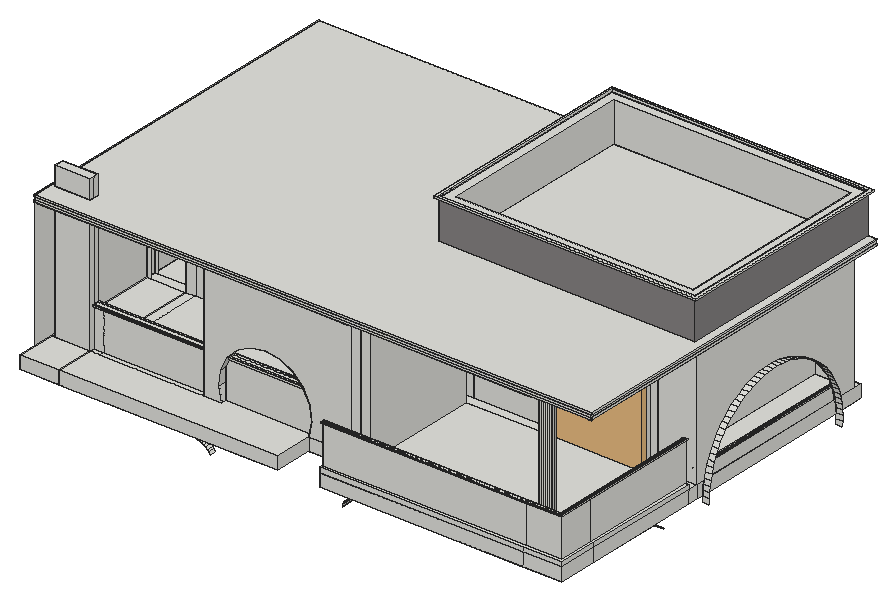
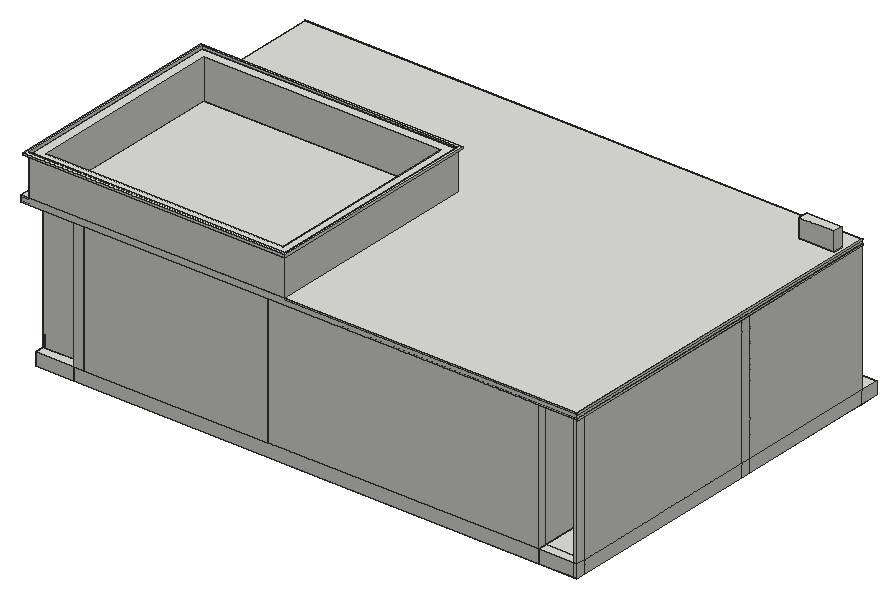
# SketchUp Ruby script. Lengths in inches.
U = 1.inch
M = Sketchup.active_model
def pt(a) = Geom::Point3d.new(a.map { |v| v * U })
def face(e, loops, mat)
  f = e.add_face(loops[0].map { |a| pt(a) })
  loops[1..].each { |l| e.add_face(l.map { |a| pt(a) }).erase! }
  f.material = f.back_material = mat if mat
  f
end
# faces: each face lists its corners as indices into pts; further lists are holes
def faces(e, pts, list, mat = nil) = list.each { |f| face(e, (f[0].is_a?(Array) ? f : [f]).map { |l| l.map { |i| pts[i] } }, mat) }
# xy, xz, yz: faces in a plane at the given z, y or x. An outline is a flat list of corners, or four numbers for a rectangle; further outlines are holes
def ring(l) = l.size == 4 ? [[l[0], l[1]], [l[2], l[1]], [l[2], l[3]], [l[0], l[3]]] : l.each_slice(2).to_a
def flat(e, list, mat, &to3) = list.each { |f| face(e, (f[0].is_a?(Array) ? f : [f]).map { |l| ring(l).map { |u, v| to3.(u, v) } }, mat) }
def xy(e, z, list, mat = nil) = flat(e, list, mat) { |x, y| [x, y, z] }
def xz(e, y, list, mat = nil) = flat(e, list, mat) { |x, z| [x, y, z] }
def yz(e, x, list, mat = nil) = flat(e, list, mat) { |y, z| [x, y, z] }
def lines(e, pts, list) = list.each { |a, b| e.add_line(pt(pts[a]), pt(pts[b])) }
# prism: a flat outline (further loops are holes) pulled along v
def prism(e, loops, v, mat = nil)
  f = face(e, loops, mat); d = Geom::Vector3d.new(v.map { |x| x * U })
  f.pushpull(f.normal.samedirection?(d) ? d.length : -d.length)
end
def box(e, o, s, mat = nil) = prism(e, [[o, [o[0] + s[0], o[1], o[2]], [o[0] + s[0], o[1] + s[1], o[2]], [o[0], o[1] + s[1], o[2]]]], [0, 0, s[2]], mat)
def at(x, y, z, deg = 0) = Geom::Transformation.translation(pt([x, y, z])) * Geom::Transformation.rotation(ORIGIN, Z_AXIS, deg.degrees)
def axes(o, x, y, z) = Geom::Transformation.new([*x, 0, *y, 0, *z, 0, *pt(o).to_a, 1])
def part(name) = M.definitions.add(name)
# library, detail: a bought-in or finely detailed component or shape, given as its bounding box
def library(name, o, s) = part(name).tap { |d| box(d.entities, o, s) }
def detail(e, o, s) = box(e.add_group.entities, o, s)
def put(e, d, t, mat = nil) = e.add_instance(d, t).tap { |i| i.material = mat if mat }
def group(e, t, mat = nil) = e.add_group.tap { |g| g.transformation = t; g.material = mat if mat }.entities
root = M.entities
M.materials.add("[Brick Tumbled]").color = [135, 132, 132]
c1 = library("Window 46-47",[-61.02,-2.17,0],[122.04,4.34,74.02])
xy(root,246,[[9,12,45,25.8125],[45,12,54,25.8125],[54,12,54,25.8125,95.3125,25.8125,95.3125,31.1875,54,31.1875,54,48,131,48,131,17.48,95.3125,17.48,95.3125,12],[95.3125,12,131,17.48],[131,12,170.0625,17.48],
  [170.0625,12,209.125,17.48],[209.125,12,248.5625,48],[317.15,12,317.15,21.82,288,21.82,288,48,477,48,477,12],[308.6875,12,317.15,21.82],[[477,12,513,48],[493.53,20.08,494.44,20.12,495.3125,20.39,496.09,20.88,496.7,21.55,497.125,22.36,497.33,23.25,497.29,24.17,497.01,25.04,496.52,25.8125,495.85,26.43,495.04,26.85,494.15,27.05,493.24,27.01,492.37,26.74,491.59,26.25,490.98,25.58,490.55,24.77,490.35,23.875,490.39,22.96,490.67,22.09,491.16,21.32,491.83,20.7,492.64,20.28]],
  [131,17.48,209.125,48],[9,25.8125,45,31.1875],[45,25.8125,54,31.1875],[9,31.1875,45,48],[45,31.1875,54,48],
  [9,48,45,57],[45,48,54,57],[54,48,288,57],[288,48,297,57],[297,48,477,57],
  [477,48,513,57],[9,57,45,351],[45,57,54,351],[54,57,288,351],[288,57,297,351],
  [297,57,468,351],[468,57,468,351,477,351,477,168.3125,472.375,168.3125,472.375,159.3125,477,159.3125,477,57],[477,57,477,159.3125,507.74,159.3125,507.74,112.49,513,112.49,513,57],[507.74,112.49,513,134.0625],[507.74,134.0625,507.74,159.3125,477,159.3125,477,168.3125,513,168.3125,513,134.0625],
  [472.375,159.3125,477,168.3125],[477,168.3125,513,351],[9,351,45,360],[45,351,288,360],[288,351,297,360],
  [297,351,477,360],[477,351,513,360]])
xy(root,258,[[9,12,45,48],[45,12,248.5625,12,248.5625,52.5,167.375,52.5,167.375,48,45,48],[288,12,288,19.75,505.25,19.75,505.25,159.3125,513,159.3125,513,12],[[288,19.75,505.25,19.75,505.25,159.3125,477,159.3125,477,48,288,48],[479.86,29.71,478.33,30.04,476.93,30.76,475.77,31.81,474.92,33.12,474.44,34.61,474.36,36.18,474.69,37.71,475.41,39.1,476.46,40.26,477.77,41.11,479.26,41.59,480.83,41.67,482.36,41.34,483.75,40.63,484.91,39.58,485.76,38.26,486.25,36.77,486.32,35.21,486,33.68,485.28,32.28,484.23,31.12,482.92,30.27,481.42,29.79]],[479.86,29.71,478.33,30.04,476.93,30.76,475.77,31.81,474.92,33.12,474.44,34.61,474.36,36.18,474.69,37.71,475.41,39.1,476.46,40.26,477.77,41.11,479.26,41.59,480.83,41.67,482.36,41.34,483.75,40.63,484.91,39.58,485.76,38.26,486.25,36.77,486.32,35.21,486,33.68,485.28,32.28,484.23,31.12,482.92,30.27,481.42,29.79],
  [9,48,12.34,57],[12.34,48,45,57],[45,48,54,52.5],[54,48,151.375,52.5],[151.375,48,167.375,57],
  [248.5625,48,297,57],[297,48,306,159.3125],[306,48,477,48,477,159.3125,469.61,159.3125,469.61,168.3125,386.17,168.3125,386.17,159.3125,306,159.3125],[45,52.5,54,57],[54,52.5,151.375,57],
  [167.375,52.5,248.5625,57],[9,57,45,159.3125],[45,57,54,159.3125],[54,57,297,159.3125],[9,159.3125,45,168.3125],
  [45,159.3125,297,168.3125],[297,159.3125,386.17,168.3125],[469.61,159.3125,477,168.3125],[477,159.3125,513,168.3125],[9,168.3125,45,351],
  [45,168.3125,54,351],[54,168.3125,297,351],[297,168.3125,297,360,468,360,468,351,306,351,306,168.3125],[306,168.3125,468,351],[468,168.3125,477,360],
  [477,168.3125,509.57,351],[[509.57,168.3125,513,351],[510.66,169.41,511.91,349.91]],[510.66,169.41,511.91,349.91],[9,351,45,360],[45,351,297,360],
  [477,351,513,360]])
xy(root,262.3125,[[288,12,513,12,513,159.3125,510.03,159.3125,510.03,14.97,288,14.97],[288,14.97,288,16.78,508.22,16.78,508.22,159.3125,510.03,159.3125,510.03,14.97],[288,16.78,508.22,16.78,508.22,159.3125,505.25,159.3125,505.25,19.75,288,19.75]])
xy(root,270.75,[[[509.78,168.53,512.79,350.79],[510.66,169.41,511.91,349.91]],[510.66,169.41,511.91,349.91]])
xy(root,271.125,[[[509.78,168.53,512.79,350.79],[510.66,169.41,511.91,349.91]],[510.66,169.41,511.91,349.91]])
xy(root,294,[[[165.34,50.46,250.6,59.04],[167.375,52.5,248.5625,57]],[[43.21,50.71,153.16,58.79],[45,52.5,151.375,57]],[45,52.5,151.375,57],[167.375,52.5,248.5625,57]])
xy(root,295.125,[[[43.21,50.71,153.16,58.79],[45,52.5,151.375,57]],[45,52.5,151.375,57]])
xy(root,295.875,[[[165.34,50.46,250.6,59.04],[167.375,52.5,248.5625,57]],[167.375,52.5,248.5625,57]])
xy(root,298.3125,[[[286.96,13.93,286.96,17.82,507.18,17.82,507.18,160.35,511.07,160.35,511.07,13.93],[288,14.97,510.03,14.97,510.03,159.3125,508.22,159.3125,508.22,16.78,288,16.78]],[288,14.97,288,16.78,508.22,16.78,508.22,159.3125,510.03,159.3125,510.03,14.97]])
xy(root,298.9375,[[[286.96,13.93,511.07,13.93,511.07,160.35,507.18,160.35,507.18,17.82,286.96,17.82],[288,14.97,288,16.78,508.22,16.78,508.22,159.3125,510.03,159.3125,510.03,14.97]],[288,14.97,510.03,14.97,510.03,159.3125,508.22,159.3125,508.22,16.78,288,16.78]])
xy(root,361.875,[[386.17,159.3125,469.61,168.3125]])
xy(root,378,[[8.375,28.625,9,29.25],[9,28.625,12.34,29.25],[12.34,28.625,151.375,29.25],[151.375,28.625,288,29.25],[288,28.625,297,29.25],
  [297,28.625,306,29.25],[306,28.625,468,29.25],[468,28.625,477,29.25],[477,28.625,526.4375,29.25],[526.4375,28.625,527.0625,29.25],
  [8.375,29.25,9,159.3125],[9,29.25,12.34,159.3125],[12.34,29.25,12.34,159.3125,297,159.3125,297,57,151.375,57,151.375,29.25],[151.375,29.25,288,48],[288,29.25,297,48],
  [297,29.25,306,48],[[306,29.25,468,159.3125],[331.16,57.35,457.66,126.29]],[468,29.25,468,159.3125,477,159.3125,477,40.61,476.46,40.26,475.41,39.1,474.69,37.71,474.36,36.18,474.44,34.61,474.92,33.12,475.77,31.81,476.93,30.76,477,30.72,477,29.25],[477,29.25,477,30.72,478.33,30.04,479.86,29.71,481.42,29.79,482.92,30.27,484.23,31.12,485.28,32.28,486,33.68,486.32,35.21,486.25,36.77,485.76,38.26,484.91,39.58,483.75,40.63,482.36,41.34,480.83,41.67,479.26,41.59,477.77,41.11,477,40.61,477,159.3125,526.4375,159.3125,526.4375,29.25],[526.4375,29.25,527.0625,159.3125],
  [479.86,29.71,481.42,29.79,482.92,30.27,484.23,31.12,485.28,32.28,486,33.68,486.32,35.21,486.25,36.77,485.76,38.26,484.91,39.58,483.75,40.63,482.36,41.34,480.83,41.67,479.26,41.59,477.77,41.11,477,40.61,477,30.72,478.33,30.04],[477,30.72,477,40.61,476.46,40.26,475.41,39.1,474.69,37.71,474.36,36.18,474.44,34.61,474.92,33.12,475.77,31.81,476.93,30.76],[151.375,48,297,57],[297,48,306,159.3125],[8.375,159.3125,9,168.3125],
  [9,159.3125,12.34,168.3125],[12.34,159.3125,45,168.3125],[45,159.3125,297,168.3125],[297,159.3125,468,168.3125],[468,159.3125,477,168.3125],
  [477,159.3125,519.125,168.3125],[519.125,159.3125,526.4375,168.3125],[526.4375,159.3125,527.0625,168.3125],[8.375,168.3125,9,351],[9,168.3125,12.34,351],
  [12.34,168.3125,45,351],[45,168.3125,54,351],[54,168.3125,297,351],[297,168.3125,297,360,468,360,468,351,306,351,306,168.3125],[306,168.3125,468,351],
  [468,168.3125,477,360],[477,168.3125,513,351],[513,168.3125,513,351,477,351,477,360,519.125,360,519.125,168.3125],[519.125,168.3125,526.4375,360],[526.4375,168.3125,527.0625,360],
  [8.375,351,9,360],[9,351,12.34,360],[12.34,351,45,360],[45,351,297,360]])
xy(root,379.5,[[8.375,28.625,9,29.25],[9,28.625,526.4375,29.25],[526.4375,28.625,527.0625,29.25],[8.375,29.25,9,360],[[9,29.25,526.4375,29.25,526.4375,360,519.25,360,519.25,158.6875,281.0625,158.6875,281.0625,360,9,360],[331.16,57.35,457.66,126.29]],
  [526.4375,29.25,527.0625,360]])
xy(root,382.75,[[8.375,28.625,9,29.25],[9,28.625,526.4375,29.25],[526.4375,28.625,527.0625,29.25],[8.375,29.25,9,360],[526.4375,29.25,527.0625,360]])
xy(root,384,[[8.375,28.625,9,29.25],[9,28.625,527.0625,29.25],[8.375,29.25,9,360],[[9,29.25,527.0625,29.25,527.0625,360,519.25,360,519.25,158.6875,281.0625,158.6875,281.0625,360,9,360],[12.34,48,45,57]],[[281.0625,158.6875,519.25,360],[289.94,167.6875,510.25,351]],
  [289.94,167.6875,510.25,351]])
xy(root,401.375,[[12.34,48,45,57]])
xy(root,420,[[[278.28,155.9,522.04,362.79],[281.0625,158.6875,519.25,360]],[[281.0625,158.6875,519.25,360],[289.94,167.6875,510.25,351]]])
xy(root,422.0625,[[[278.28,155.9,522.04,362.79],[281.0625,158.6875,519.25,360]]])
xz(root,12,[[9,246,45,258],[45,246,248.5625,258],[288,246,477,258],[477,246,513,258],[288,258,477,262.3125],
  [477,258,513,262.3125]])
xz(root,13.93,[[286.96,298.3125,477,298.9375],[477,298.3125,511.07,298.9375]])
xz(root,14.97,[[288,262.3125,477,298.3125],[477,262.3125,510.03,298.3125],[288,298.3125,477,298.9375],[477,298.3125,510.03,298.9375]])
xz(root,16.78,[[288,262.3125,477,298.3125],[477,262.3125,508.22,298.3125],[288,298.3125,477,298.9375],[477,298.3125,508.22,298.9375]])
xz(root,17.82,[[286.96,298.3125,477,298.9375],[477,298.3125,507.18,298.9375]])
xz(root,19.75,[[288,258,477,262.3125],[477,258,505.25,262.3125]])
xz(root,28.625,[[8.375,378,9,379.5],[9,378,526.4375,379.5],[526.4375,378,527.0625,379.5],[8.375,382.75,9,384],[9,382.75,527.0625,384]])
xz(root,29.25,[[8.375,378,9,379.5],[9,378,526.4375,379.5],[526.4375,378,527.0625,379.5],[9,379.5,526.4375,382.75],[8.375,382.75,9,384],
  [9,382.75,527.0625,384]])
xz(root,48,[[248.5625,246,288,258],[288,246,477,258],[12.34,258,45,384],[151.375,258,167.375,258,164.87,271.46,166.72,285.03,172.72,297.34,182.29,307.14,194.45,313.45,207.97,315.625,221.49,313.45,233.65,307.14,243.21,297.34,249.22,285.03,251.07,271.46,248.5625,258,288,258,288,378,151.375,378],[288,258,297,378],
  [297,258,306,378],[12.34,384,45,401.375]])
xz(root,50.46,[[165.34,294,250.6,295.875]])
xz(root,50.71,[[43.21,294,54,295.125],[54,294,153.16,295.125]])
xz(root,52.5,[[45,258,54,294],[54,258,151.375,294],[167.375,258,248.5625,294],[45,294,54,295.125],[54,294,151.375,295.125],
  [167.375,294,248.5625,295.875]])
xz(root,57,[[12.34,258,45,384],[45,258,54,294],[54,258,151.375,294],[151.375,258,151.375,378,297,378,297,258,248.5625,258,251.07,271.46,249.22,285.03,248.5625,286.38,248.5625,295.875,243.93,295.875,243.21,297.34,233.65,307.14,221.49,313.45,207.97,315.625,194.45,313.45,182.29,307.14,172.72,297.34,172.01,295.875,167.375,295.875,167.375,286.38,166.72,285.03,164.87,271.46,167.375,258],[167.375,258,167.375,286.38,171.09,294,244.84,294,248.5625,286.38,248.5625,258],
  [167.375,286.38,167.375,294,171.09,294],[248.5625,286.38,244.84,294,248.5625,294],[45,294,54,295.125],[54,294,151.375,295.125],[167.375,294,171.09,295.875],
  [171.09,294,172.01,295.875,171.09,295.875],[171.09,294,244.84,294,243.93,295.875,172.01,295.875],[244.84,294,244.84,295.875,243.93,295.875],[244.84,294,248.5625,295.875],[12.34,384,45,401.375]])
xz(root,57.35,[[331.16,378,457.66,379.5]])
xz(root,58.79,[[43.21,294,54,295.125],[54,294,153.16,295.125]])
xz(root,59.04,[[165.34,294,171.09,295.875],[171.09,294,244.84,295.875],[244.84,294,250.6,295.875]])
xz(root,126.29,[[331.16,378,457.66,379.5]])
xz(root,155.9,[[278.28,420,522.04,422.0625]])
xz(root,158.6875,[[281.0625,420,519.25,422.0625]])
xz(root,158.6875,[[281.0625,384,519.25,420]],"[Brick Tumbled]")
xz(root,159.3125,[[9,258,12.34,378],[45,258,54,378],[54,258,297,378],[297,258,306,378],[505.25,258,513,262.3125],
  [508.22,262.3125,510.03,298.3125],[508.22,298.3125,510.03,298.9375]])
xz(root,160.35,[[507.18,298.3125,511.07,298.9375]])
xz(root,167.6875,[[289.94,384,510.25,420]])
xz(root,168.3125,[[9,258,12.34,378],[45,258,54,378],[54,258,297,378],[297,258,306,378],[306,258,306,378,468,378,468,361.875,386.17,361.875,386.17,258],
  [468,258,469.61,361.875],[469.61,258,469.61,361.875,468,361.875,468,378,477,378,477,258],[477,258,513,378]])
xz(root,168.53,[[509.78,270.75,512.79,271.125]])
xz(root,169.41,[[510.66,258,511.91,270.75],[510.66,270.75,511.91,271.125]])
xz(root,349.91,[[510.66,258,511.91,270.75],[510.66,270.75,511.91,271.125]])
xz(root,350.79,[[509.78,270.75,512.79,271.125]])
xz(root,351,[[9,246,12.34,258],[9,258,12.34,378],[45,258,54,378],[54,258,297,378],[306,258,468,378],
  [477,258,513,378],[289.94,384,510.25,420]])
xz(root,360,[[9,246,12.34,258],[12.34,246,45,258],[45,246,477,258],[477,246,513,258],[9,258,12.34,378],
  [45,258,297,378],[297,258,468,378],[468,258,477,378],[8.375,378,9,379.5],[9,378,9,384,527.0625,384,527.0625,382.75,526.4375,382.75,526.4375,378],
  [526.4375,378,527.0625,379.5],[8.375,382.75,9,384],[281.0625,384,519.25,420],[281.0625,420,519.25,422.0625]])
xz(root,362.79,[[278.28,420,522.04,422.0625]])
yz(root,8.375,[[28.625,378,29.25,379.5],[29.25,378,360,379.5],[28.625,382.75,29.25,384],[29.25,382.75,360,384]])
yz(root,9,[[12,246,29.25,258],[29.25,246,159.3125,258],[159.3125,246,168.3125,258],[168.3125,246,351,258],[351,246,360,258],
  [29.25,258,159.3125,378],[159.3125,258,168.3125,378],[168.3125,258,351,378],[351,258,360,378],[28.625,378,29.25,379.5],
  [29.25,378,360,379.5],[29.25,379.5,360,382.75],[28.625,382.75,29.25,384],[29.25,382.75,360,384]])
yz(root,12.34,[[48,258,57,378],[48,378,57,384],[48,384,57,401.375]])
yz(root,43.21,[[50.71,294,58.79,295.125]])
yz(root,45,[[12,246,360,258],[48,258,52.5,384],[52.5,258,57,294],[159.3125,258,168.3125,378],[168.3125,258,351,378],
  [351,258,360,378],[52.5,294,57,295.125],[52.5,295.125,57,384],[48,384,52.5,401.375],[52.5,384,57,401.375]])
yz(root,54,[[168.3125,258,351,378]])
yz(root,151.375,[[48,258,48,378,57,378,57,295.125,52.5,295.125,52.5,258],[52.5,258,57,294],[52.5,294,57,295.125]])
yz(root,153.16,[[50.71,294,58.79,295.125]])
yz(root,165.34,[[50.46,294,59.04,295.875]])
yz(root,167.375,[[52.5,258,57,294],[52.5,294,57,295.875]])
yz(root,248.5625,[[12,246,48,258],[52.5,258,57,294],[52.5,294,57,295.875]])
yz(root,250.6,[[50.46,294,59.04,295.875]])
yz(root,278.28,[[155.9,420,362.79,422.0625]])
yz(root,281.0625,[[158.6875,384,360,420],[158.6875,420,360,422.0625]])
yz(root,286.96,[[13.93,298.3125,17.82,298.9375]])
yz(root,288,[[12,246,48,258],[12,258,19.75,262.3125],[14.97,262.3125,16.78,298.3125],[14.97,298.3125,16.78,298.9375]])
yz(root,289.94,[[167.6875,384,351,420]])
yz(root,297,[[48,258,57,378],[57,258,159.3125,378],[159.3125,258,168.3125,378],[168.3125,258,351,378],[351,258,360,378]])
yz(root,306,[[48,258,159.3125,378],[168.3125,258,351,378]])
yz(root,331.16,[[57.35,378,126.29,379.5]])
yz(root,386.17,[[159.3125,258,168.3125,361.875]])
yz(root,457.66,[[57.35,378,126.29,379.5]])
yz(root,468,[[168.3125,258,351,378],[351,258,360,378]])
yz(root,469.61,[[159.3125,258,168.3125,361.875]])
yz(root,477,[[48,246,360,258],[168.3125,258,351,378]])
yz(root,505.25,[[19.75,258,48,262.3125],[48,258,159.3125,262.3125]])
yz(root,507.18,[[17.82,298.3125,48,298.9375],[48,298.3125,160.35,298.9375]])
yz(root,508.22,[[16.78,262.3125,48,298.3125],[48,262.3125,159.3125,298.3125],[16.78,298.3125,48,298.9375],[48,298.3125,159.3125,298.9375]])
yz(root,509.78,[[168.53,270.75,176.75,271.125],[176.75,270.75,329.3125,271.125],[329.3125,270.75,350.79,271.125]])
yz(root,510.03,[[14.97,262.3125,48,298.3125],[48,262.3125,159.3125,298.3125],[14.97,298.3125,48,298.9375],[48,298.3125,159.3125,298.9375]])
yz(root,510.25,[[167.6875,384,351,420]])
yz(root,510.66,[[169.41,258,176.75,270.75],[176.75,258,329.3125,270.75],[329.3125,258,349.91,270.75],[169.41,270.75,176.75,271.125],[176.75,270.75,329.3125,271.125],
  [329.3125,270.75,349.91,271.125]])
yz(root,511.07,[[13.93,298.3125,48,298.9375],[48,298.3125,160.35,298.9375]])
yz(root,511.91,[[169.41,258,176.75,270.75],[176.75,258,329.3125,270.75],[329.3125,258,349.91,270.75],[169.41,270.75,176.75,271.125],[176.75,270.75,329.3125,271.125],
  [329.3125,270.75,349.91,271.125]])
yz(root,512.79,[[168.53,270.75,176.75,271.125],[176.75,270.75,329.3125,271.125],[329.3125,270.75,350.79,271.125]])
yz(root,513,[[12,246,48,258],[48,246,159.3125,258],[159.3125,246,168.3125,258],[168.3125,246,175.45,246,175.67,250.33,176.24,255.18,176.75,258,168.3125,258],[175.45,246,330.59,246,330.58,247.04,330.23,251.91,329.57,256.74,329.3125,258,176.75,258,176.24,255.18,175.67,250.33],
  [330.59,246,360,246,360,258,329.3125,258,329.57,256.74,330.23,251.91,330.58,247.04],[12,258,48,262.3125],[48,258,159.3125,262.3125],[168.3125,258,168.3125,378,351,378,351,258,329.3125,258,328.6,261.52,327.34,266.23,325.79,270.85,323.95,275.37,321.83,279.76,319.43,284.01,316.78,288.1,313.87,292.01,310.73,295.74,307.35,299.26,303.76,302.5625,299.97,305.63,296,308.46,291.86,311.03,287.56,313.33,283.125,315.37,278.57,317.12,273.92,318.57,269.1875,319.74,264.39,320.6,259.54,321.17,254.67,321.42,249.8,321.37,244.93,321.02,240.1,320.36,235.32,319.39,230.61,318.13,225.99,316.58,221.47,314.74,217.08,312.62,212.83,310.22,208.74,307.57,204.83,304.66,201.1,301.52,197.58,298.14,194.28,294.55,191.21,290.76,188.38,286.79,185.8125,282.65,183.51,278.35,181.47,273.92,179.73,269.36,178.27,264.71,177.1,259.98,176.75,258]])
yz(root,519.25,[[158.6875,420,360,422.0625]])
yz(root,519.25,[[158.6875,384,360,420]],"[Brick Tumbled]")
yz(root,522.04,[[155.9,420,362.79,422.0625]])
yz(root,526.4375,[[28.625,378,29.25,379.5],[29.25,378,360,379.5],[29.25,379.5,360,382.75]])
yz(root,527.0625,[[28.625,378,29.25,379.5],[29.25,378,360,379.5],[28.625,382.75,29.25,384],[29.25,382.75,360,384]])
p = [[308.96,12,237.7],[308.76,12,236.49],[308.76,21.82,236.49],[308.96,21.82,237.7],[185.98,12,236.95],[184.79,12,238.71],
  [184.79,17.48,238.71],[185.98,17.48,236.95],[519.125,330.375,237.3],[519.125,330.63,242.17],[513,330.63,242.17],[513,330.375,237.3],
  [513,130.5,237.57],[513,128.95,239.25],[507.74,128.95,239.25],[507.74,130.5,237.57],[309.3,12,238.88],[309.3,21.82,238.88],
  [183.41,12,240.33],[183.41,17.48,240.33],[309.76,12,240.02],[309.76,21.82,240.02],[513,127.25,240.77],[507.74,127.25,240.77],
  [310.35,12,241.1],[310.35,21.82,241.1],[181.84,12,241.77],[181.84,17.48,241.77],[519.125,175.42,245.46],[519.125,175.47,240.59],
  [513,175.47,240.59],[513,175.42,245.46],[513,125.41,242.12],[507.74,125.41,242.12],[311.06,12,242.1],[311.06,21.82,242.1],
  [180.13,12,243.03],[180.13,17.48,243.03],[311.87,12,243.02],[311.87,21.82,243.02],[513,123.45,243.28],[507.74,123.45,243.28],
  [519.125,330.58,247.04],[513,330.58,247.04],[513,330.59,246],[178.28,12,244.08],[178.28,17.48,244.08],[312.78,12,243.85],
  [312.78,21.82,243.85],[513,121.38,244.25],[507.74,121.38,244.25],[313.77,12,244.5625],[313.77,21.82,244.5625],[176.32,12,244.91],
  [176.32,17.48,244.91],[513,119.23,245.01],[507.74,119.23,245.01],[314.84,12,245.17],[314.84,21.82,245.17],[174.28,12,245.51],
  [174.28,17.48,245.51],[513,117.02,245.56],[507.74,117.02,245.56],[315.97,12,245.65],[315.97,21.82,245.65],[172.1875,12,245.88],
  [172.1875,17.48,245.88],[519.125,175.67,250.33],[513,175.45,246],[513,175.67,250.33],[317.15,12,246],[317.15,21.82,246],
  [513,114.76,245.89],[507.74,114.76,245.89],[170.0625,12,246],[170.0625,17.48,246],[513,112.49,246],[507.74,112.49,246],
  [519.125,330.23,251.91],[513,330.23,251.91],[519.125,176.24,255.18],[513,176.24,255.18],[519.125,329.57,256.74],[513,329.57,256.74],
  [519.125,177.1,259.98],[513,176.75,258],[513,177.1,259.98],[519.125,328.6,261.52],[513,328.6,261.52],[513,329.3125,258],
  [478.33,30.04,258],[479.86,29.71,258],[479.86,29.71,378],[478.33,30.04,378],[481.42,29.79,258],[481.42,29.79,378],
  [482.92,30.27,258],[482.92,30.27,378],[476.93,30.76,258],[477,30.72,378],[476.93,30.76,378],[484.23,31.12,258],
  [484.23,31.12,378],[475.77,31.81,258],[475.77,31.81,378],[485.28,32.28,258],[485.28,32.28,378],[474.92,33.12,258],
  [474.92,33.12,378],[486,33.68,258],[486,33.68,378],[474.44,34.61,258],[474.44,34.61,378],[486.32,35.21,258],
  [486.32,35.21,378],[474.36,36.18,258],[474.36,36.18,378],[486.25,36.77,258],[486.25,36.77,378],[474.69,37.71,258],
  [474.69,37.71,378],[485.76,38.26,258],[485.76,38.26,378],[475.41,39.1,258],[475.41,39.1,378],[484.91,39.58,258],
  [484.91,39.58,378],[476.46,40.26,258],[476.46,40.26,378],[483.75,40.63,258],[483.75,40.63,378],[477.77,41.11,258],
  [477,40.61,378],[477.77,41.11,378],[482.36,41.34,258],[482.36,41.34,378],[479.26,41.59,258],[479.26,41.59,378],
  [480.83,41.67,258],[480.83,41.67,378],[164.87,48,271.46],[167.375,48,258],[167.375,52.5,258],[167.375,57,258],
  [164.87,57,271.46],[248.5625,48,258],[251.07,48,271.46],[251.07,57,271.46],[248.5625,57,258],[248.5625,52.5,258],
  [519.125,178.27,264.71],[513,178.27,264.71],[519.125,327.34,266.23],[513,327.34,266.23],[519.125,179.73,269.36],[513,179.73,269.36],
  [519.125,325.79,270.85],[513,325.79,270.85],[519.125,181.47,273.92],[513,181.47,273.92],[519.125,323.95,275.37],[513,323.95,275.37],
  [166.72,48,285.03],[166.72,57,285.03],[249.22,48,285.03],[249.22,57,285.03],[519.125,183.51,278.35],[513,183.51,278.35],
  [519.125,321.83,279.76],[513,321.83,279.76],[519.125,185.8125,282.65],[513,185.8125,282.65],[519.125,319.43,284.01],[513,319.43,284.01],
  [519.125,188.38,286.79],[513,188.38,286.79],[519.125,316.78,288.1],[513,316.78,288.1],[172.72,48,297.34],[167.375,57,286.38],
  [171.09,57,294],[172.01,57,295.875],[172.72,57,297.34],[243.21,48,297.34],[243.21,57,297.34],[243.93,57,295.875],
  [244.84,57,294],[248.5625,57,286.38],[519.125,191.21,290.76],[513,191.21,290.76],[519.125,313.87,292.01],[513,313.87,292.01],
  [519.125,194.28,294.55],[513,194.28,294.55],[519.125,310.73,295.74],[513,310.73,295.74],[519.125,197.58,298.14],[513,197.58,298.14],
  [519.125,307.35,299.26],[513,307.35,299.26],[182.29,48,307.14],[182.29,57,307.14],[233.65,48,307.14],[233.65,57,307.14],
  [519.125,201.1,301.52],[513,201.1,301.52],[519.125,303.76,302.5625],[513,303.76,302.5625],[519.125,204.83,304.66],[513,204.83,304.66],
  [519.125,299.97,305.63],[513,299.97,305.63],[519.125,208.74,307.57],[513,208.74,307.57],[519.125,296,308.46],[513,296,308.46],
  [194.45,48,313.45],[194.45,57,313.45],[221.49,48,313.45],[221.49,57,313.45],[519.125,212.83,310.22],[513,212.83,310.22],
  [519.125,291.86,311.03],[513,291.86,311.03],[519.125,217.08,312.62],[513,217.08,312.62],[519.125,287.56,313.33],[513,287.56,313.33],
  [519.125,221.47,314.74],[513,221.47,314.74],[519.125,283.125,315.37],[513,283.125,315.37],[207.97,48,315.625],[207.97,57,315.625],
  [519.125,225.99,316.58],[513,225.99,316.58],[519.125,278.57,317.12],[513,278.57,317.12],[519.125,230.61,318.13],[513,230.61,318.13],
  [519.125,273.92,318.57],[513,273.92,318.57],[519.125,235.32,319.39],[513,235.32,319.39],[519.125,269.1875,319.74],[513,269.1875,319.74],
  [519.125,240.1,320.36],[513,240.1,320.36],[519.125,264.39,320.6],[513,264.39,320.6],[519.125,244.93,321.02],[513,244.93,321.02],
  [519.125,259.54,321.17],[513,259.54,321.17],[519.125,249.8,321.37],[513,249.8,321.37],[519.125,254.67,321.42],[513,254.67,321.42],
  [519.25,360,382.75],[519.25,158.6875,382.75],[281.0625,158.6875,382.75],[281.0625,360,382.75],[526.4375,360,382.75],[9,360,382.75]]
faces(root,p,[[0,1,2,3],[4,5,6,7],[8,9,10,11],[12,13,14,15],[16,0,3,17],[5,18,19,6],[20,16,17,21],[13,22,23,14],
  [24,20,21,25],[18,26,27,19],[28,29,30,31],[22,32,33,23],[34,24,25,35],[26,36,37,27],[38,34,35,39],[32,40,41,33],
  [9,42,43,44,10],[36,45,46,37],[47,38,39,48],[40,49,50,41],[51,47,48,52],[45,53,54,46],[49,55,56,50],[57,51,52,58],
  [53,59,60,54],[55,61,62,56],[63,57,58,64],[59,65,66,60],[67,28,31,68,69],[70,63,64,71],[61,72,73,62],[65,74,75,66],
  [72,76,77,73],[42,78,79,43],[80,67,69,81],[78,82,83,79],[84,80,81,85,86],[82,87,88,89,83],[90,91,92,93],[91,94,95,92],
  [94,96,97,95],[98,90,93,99,100],[96,101,102,97],[103,98,100,104],[101,105,106,102],[107,103,104,108],[105,109,110,106],[111,107,108,112],
  [109,113,114,110],[115,111,112,116],[113,117,118,114],[119,115,116,120],[117,121,122,118],[123,119,120,124],[121,125,126,122],[127,123,124,128],
  [125,129,130,126],[131,127,128,132,133],[129,134,135,130],[136,131,133,137],[134,138,139,135],[138,136,137,139],[140,141,142,143,144],[145,146,147,148,149],
  [150,84,86,151],[87,152,153,88],[154,150,151,155],[152,156,157,153],[158,154,155,159],[156,160,161,157],[162,140,144,163],[146,164,165,147],
  [166,158,159,167],[160,168,169,161],[170,166,167,171],[168,172,173,169],[174,170,171,175],[172,176,177,173],[178,162,163,179,180,181,182],[164,183,184,185,186,187,165],
  [188,174,175,189],[176,190,191,177],[192,188,189,193],[190,194,195,191],[196,192,193,197],[194,198,199,195],[200,178,182,201],[183,202,203,184],
  [204,196,197,205],[198,206,207,199],[208,204,205,209],[206,210,211,207],[212,208,209,213],[210,214,215,211],[216,200,201,217],[202,218,219,203],
  [220,212,213,221],[214,222,223,215],[224,220,221,225],[222,226,227,223],[228,224,225,229],[226,230,231,227],[232,216,217,233],[218,232,233,219],
  [234,228,229,235],[230,236,237,231],[238,234,235,239],[236,240,241,237],[242,238,239,243],[240,244,245,241],[246,242,243,247],[244,248,249,245],
  [250,246,247,251],[248,252,253,249],[254,250,251,255],[252,256,257,253],[256,254,255,257]])
lines(root,p,[[258,259],[259,260],[260,261],[258,262],[263,261]])
put(root,c1,axes([428,161.46,257.95],[0.68195,0,0],[0,1,0],[0,0,1.40078]))
